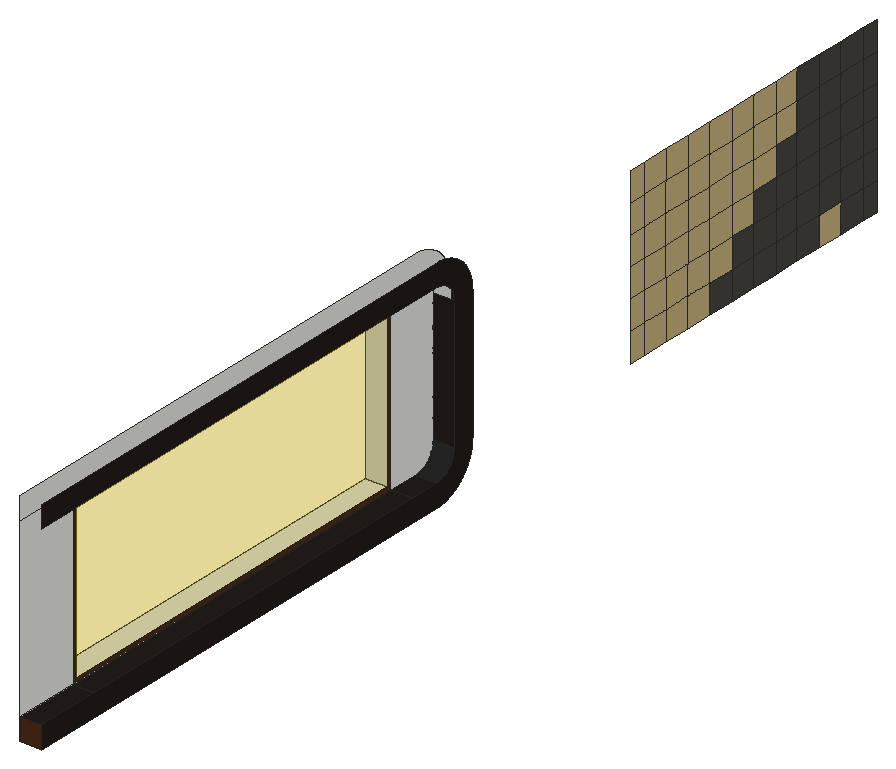
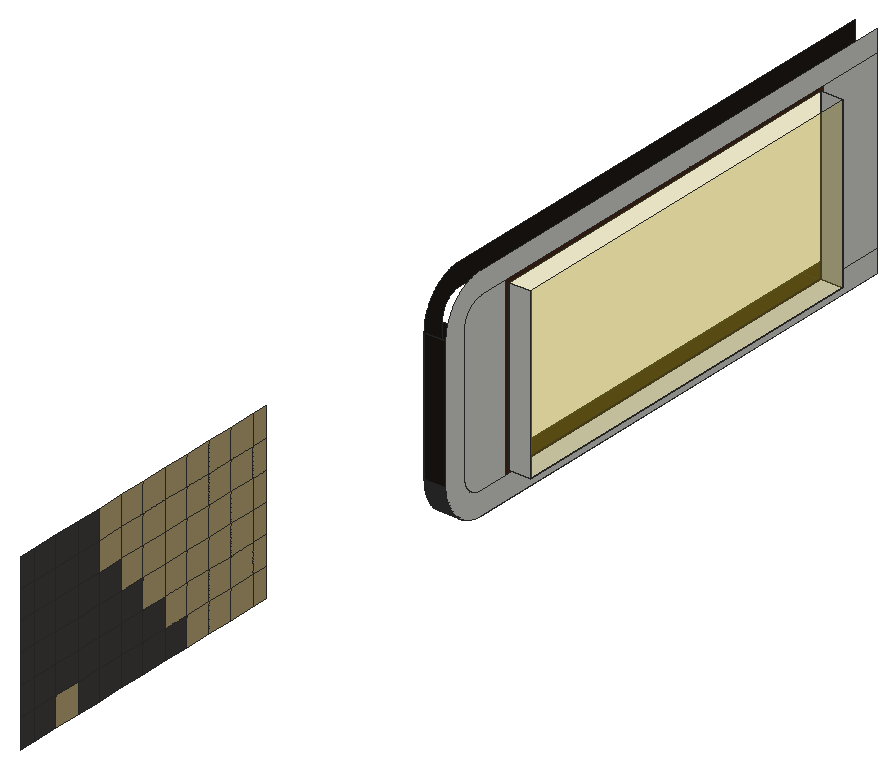
# SketchUp Ruby script. Lengths in inches.
U = 1.inch
M = Sketchup.active_model
def pt(a) = Geom::Point3d.new(a.map { |v| v * U })
def face(e, loops, mat)
  f = e.add_face(loops[0].map { |a| pt(a) })
  loops[1..].each { |l| e.add_face(l.map { |a| pt(a) }).erase! }
  f.material = f.back_material = mat if mat
  f
end
# faces: each face lists its corners as indices into pts; further lists are holes
def faces(e, pts, list, mat = nil) = list.each { |f| face(e, (f[0].is_a?(Array) ? f : [f]).map { |l| l.map { |i| pts[i] } }, mat) }
# xy, xz, yz: faces in a plane at the given z, y or x. An outline is a flat list of corners, or four numbers for a rectangle; further outlines are holes
def ring(l) = l.size == 4 ? [[l[0], l[1]], [l[2], l[1]], [l[2], l[3]], [l[0], l[3]]] : l.each_slice(2).to_a
def flat(e, list, mat, &to3) = list.each { |f| face(e, (f[0].is_a?(Array) ? f : [f]).map { |l| ring(l).map { |u, v| to3.(u, v) } }, mat) }
def xy(e, z, list, mat = nil) = flat(e, list, mat) { |x, y| [x, y, z] }
def xz(e, y, list, mat = nil) = flat(e, list, mat) { |x, z| [x, y, z] }
def yz(e, x, list, mat = nil) = flat(e, list, mat) { |y, z| [x, y, z] }
def lines(e, pts, list) = list.each { |a, b| e.add_line(pt(pts[a]), pt(pts[b])) }
# prism: a flat outline (further loops are holes) pulled along v
def prism(e, loops, v, mat = nil)
  f = face(e, loops, mat); d = Geom::Vector3d.new(v.map { |x| x * U })
  f.pushpull(f.normal.samedirection?(d) ? d.length : -d.length)
end
def box(e, o, s, mat = nil) = prism(e, [[o, [o[0] + s[0], o[1], o[2]], [o[0] + s[0], o[1] + s[1], o[2]], [o[0], o[1] + s[1], o[2]]]], [0, 0, s[2]], mat)
def at(x, y, z, deg = 0) = Geom::Transformation.translation(pt([x, y, z])) * Geom::Transformation.rotation(ORIGIN, Z_AXIS, deg.degrees)
def axes(o, x, y, z) = Geom::Transformation.new([*x, 0, *y, 0, *z, 0, *pt(o).to_a, 1])
def part(name) = M.definitions.add(name)
# library, detail: a bought-in or finely detailed component or shape, given as its bounding box
def library(name, o, s) = part(name).tap { |d| box(d.entities, o, s) }
def detail(e, o, s) = box(e.add_group.entities, o, s)
def put(e, d, t, mat = nil) = e.add_instance(d, t).tap { |i| i.material = mat if mat }
def group(e, t, mat = nil) = e.add_group.tap { |g| g.transformation = t; g.material = mat if mat }.entities
root = M.entities
M.materials.add("Glass_Basic_01").color = [255, 223, 26]
M.materials["Glass_Basic_01"].alpha = 0.25
M.materials.add("Metal_10_1K").color = [196, 175, 123]
M.materials.add("Wood_Floor_12_1K").color = [35, 29, 25]
M.materials.add("Wood_Planks_01_1K").color = [69, 67, 63]
M.materials.add("[Wood_Cherry_Original]1").color = [76, 43, 21]
xy(root,204,[[129,15,135,149.96],[129,149.96,135,150.15]],"Wood_Floor_12_1K")
xy(root,204.01,[[129,150.34,135,150.52]],"Wood_Floor_12_1K")
xy(root,210,[[129,15,135,33],[129,33,135,141.71],[129,141.71,135,149.96],[129,149.96,135,150.05],[129,150.05,135,150.15]],"Wood_Floor_12_1K")
xy(root,210.01,[[129,150.24,135,150.34]],"Wood_Floor_12_1K")
xy(root,211,[[123,34,129,140.71]])
xz(root,15,[[129,204,135,210]],"[Wood_Cherry_Original]1")
xz(root,34,[[123,211,129,257]])
xz(root,140.71,[[123,211,129,257]])
xz(root,155.95,[[129,215.625,135,215.72]],"Wood_Floor_12_1K")
xz(root,155.96,[[129,215.8125,135,215.91],[129,215.91,135,216],[129,216,135,252]],"Wood_Floor_12_1K")
xz(root,161.95,[[129,215.43,135,215.625]],"Wood_Floor_12_1K")
xz(root,161.96,[[129,215.8125,135,216],[129,216,135,252]],"Wood_Floor_12_1K")
yz(root,123,[[34,211,140.71,257]],"Glass_Basic_01")
yz(root,129,[[15,204,150.15,204,150.34,204.01,150.52,204.01,150.71,204.02,150.9,204.04,151.09,204.05,151.28,204.07,151.46,204.09,151.84,204.15,152.02,204.18,152.21,204.21,152.39,204.25,152.58,204.29,152.76,204.33,152.94,204.38,153.31,204.48,153.49,204.53,153.85,204.65,154.02,204.71,154.2,204.77,154.38,204.84,154.55,204.91,154.73,204.99,154.9,205.0625,155.07,205.14,155.24,205.22,155.41,205.31,155.57,205.39,155.74,205.48,155.91,205.58,156.07,205.67,156.55,205.97,156.7,206.08,156.86,206.18,157.16,206.4,157.3125,206.52,157.46,206.63,157.61,206.75,157.75,206.875,157.9,207,158.04,207.125,158.17,207.25,158.3125,207.38,158.44,207.51,158.58,207.65,158.71,207.79,158.84,207.92,158.96,208.0625,159.08,208.21,159.21,208.35,159.32,208.5,159.44,208.65,159.56,208.79,159.67,208.95,159.78,209.1,159.88,209.25,159.99,209.41,160.29,209.89,160.38,210.05,160.48,210.22,160.56,210.38,160.74,210.72,160.82,210.89,160.9,211.0625,160.97,211.23,161.05,211.41,161.12,211.58,161.18,211.76,161.25,211.94,161.3125,212.11,161.37,212.29,161.43,212.47,161.53,212.83,161.58,213.02,161.63,213.2,161.67,213.38,161.71,213.57,161.75,213.75,161.78,213.9375,161.8125,214.12,161.84,214.31,161.86,214.5,161.89,214.68,161.91,214.87,161.92,215.06,161.9375,215.25,161.95,215.43,161.95,215.625,161.96,215.8125,161.96,252.1875,161.95,252.375,161.95,252.57,161.9375,252.75,161.92,252.94,161.91,253.13,161.89,253.32,161.86,253.5,161.84,253.69,161.8125,253.88,161.78,254.0625,161.75,254.25,161.71,254.43,161.67,254.62,161.63,254.8,161.58,254.98,161.53,255.17,161.43,255.53,161.37,255.71,161.3125,255.89,161.25,256.06,161.18,256.24,161.12,256.42,161.05,256.59,160.97,256.77,160.9,256.9375,160.82,257.11,160.74,257.28,160.56,257.62,160.48,257.78,160.38,257.95,160.29,258.11,159.99,258.59,159.88,258.75,159.78,258.9,159.67,259.05,159.56,259.21,159.44,259.35,159.32,259.5,159.21,259.65,159.08,259.79,158.96,259.9375,158.84,260.08,158.71,260.21,158.58,260.35,158.44,260.49,158.3125,260.62,158.17,260.75,158.04,260.875,157.9,261,157.75,261.125,157.61,261.25,157.46,261.37,157.3125,261.48,157.16,261.6,156.86,261.82,156.7,261.92,156.55,262.03,156.07,262.33,155.91,262.42,155.74,262.52,155.57,262.61,155.41,262.69,155.24,262.78,155.07,262.86,154.9,262.9375,154.73,263.01,154.55,263.09,154.38,263.16,154.2,263.23,154.02,263.29,153.85,263.35,153.49,263.47,153.31,263.52,152.94,263.62,152.76,263.67,152.58,263.71,152.39,263.75,152.21,263.79,152.02,263.82,151.84,263.85,151.46,263.91,151.28,263.93,151.09,263.95,150.9,263.96,150.71,263.98,150.52,263.99,150.34,263.99,150.15,264,15,264,15,258,150.15,258,150.24,257.99,150.34,257.99,150.52,257.97,150.62,257.96,150.8,257.94,150.9,257.93,151.08,257.89,151.18,257.875,151.27,257.86,151.36,257.83,151.45,257.8125,151.54,257.79,151.72,257.73,151.8125,257.71,151.9,257.68,151.99,257.65,152.08,257.61,152.17,257.58,152.26,257.54,152.34,257.51,152.43,257.47,152.51,257.43,152.6,257.39,152.68,257.35,152.77,257.3,152.85,257.26,153.01,257.16,153.09,257.12,153.17,257.07,153.25,257.01,153.41,256.91,153.49,256.85,153.5625,256.8,153.64,256.74,153.71,256.68,153.78,256.625,153.86,256.5625,154.07,256.375,154.14,256.31,154.2,256.24,154.27,256.18,154.33,256.11,154.4,256.04,154.52,255.9,154.58,255.82,154.7,255.68,154.8125,255.53,154.87,255.45,154.97,255.29,155.03,255.21,155.08,255.13,155.17,254.97,155.22,254.89,155.26,254.81,155.31,254.72,155.35,254.64,155.39,254.55,155.43,254.47,155.47,254.38,155.5,254.3,155.54,254.21,155.6,254.03,155.64,253.94,155.67,253.85,155.69,253.76,155.75,253.58,155.79,253.4,155.82,253.31,155.83,253.22,155.87,253.03,155.89,252.9375,155.9,252.85,155.91,252.75,155.92,252.66,155.93,252.56,155.94,252.47,155.95,252.375,155.95,252.28,155.96,252.1875,155.96,215.8125,155.95,215.72,155.95,215.625,155.94,215.53,155.93,215.44,155.92,215.34,155.91,215.25,155.9,215.15,155.89,215.0625,155.87,214.97,155.83,214.78,155.82,214.69,155.79,214.6,155.75,214.42,155.69,214.24,155.67,214.15,155.64,214.06,155.6,213.97,155.54,213.79,155.5,213.7,155.47,213.62,155.43,213.53,155.39,213.45,155.35,213.36,155.31,213.28,155.26,213.19,155.22,213.11,155.17,213.03,155.08,212.87,155.03,212.79,154.97,212.71,154.87,212.55,154.8125,212.47,154.7,212.32,154.58,212.18,154.52,212.1,154.4,211.96,154.33,211.89,154.27,211.82,154.2,211.76,154.14,211.69,154.07,211.625,153.86,211.4375,153.78,211.375,153.71,211.32,153.64,211.26,153.5625,211.2,153.49,211.15,153.41,211.09,153.25,210.99,153.17,210.93,153.09,210.88,153.01,210.84,152.85,210.74,152.77,210.7,152.68,210.65,152.6,210.61,152.51,210.57,152.43,210.53,152.34,210.49,152.26,210.46,152.17,210.42,152.08,210.39,151.99,210.35,151.9,210.32,151.8125,210.29,151.72,210.27,151.54,210.21,151.45,210.1875,151.36,210.17,151.27,210.14,151.18,210.125,151.08,210.11,150.9,210.07,150.8,210.06,150.62,210.04,150.52,210.03,150.34,210.01,150.24,210.01,150.15,210,15,210],[15,210,33,258],[141.71,210,150.15,210,150.24,210.01,150.34,210.01,150.52,210.03,150.62,210.04,150.8,210.06,150.9,210.07,151.08,210.11,151.18,210.125,151.27,210.14,151.36,210.17,151.45,210.1875,151.54,210.21,151.72,210.27,151.8125,210.29,151.9,210.32,151.99,210.35,152.08,210.39,152.17,210.42,152.26,210.46,152.34,210.49,152.43,210.53,152.51,210.57,152.6,210.61,152.68,210.65,152.77,210.7,152.85,210.74,153.01,210.84,153.09,210.88,153.17,210.93,153.25,210.99,153.41,211.09,153.49,211.15,153.5625,211.2,153.64,211.26,153.71,211.32,153.78,211.375,153.86,211.4375,154.07,211.625,154.14,211.69,154.2,211.76,154.27,211.82,154.33,211.89,154.4,211.96,154.52,212.1,154.58,212.18,154.7,212.32,154.8125,212.47,154.87,212.55,154.97,212.71,155.03,212.79,155.08,212.87,155.17,213.03,155.22,213.11,155.26,213.19,155.31,213.28,155.35,213.36,155.39,213.45,155.43,213.53,155.47,213.62,155.5,213.7,155.54,213.79,155.6,213.97,155.64,214.06,155.67,214.15,155.69,214.24,155.75,214.42,155.79,214.6,155.82,214.69,155.83,214.78,155.87,214.97,155.89,215.0625,155.9,215.15,155.91,215.25,155.92,215.34,155.93,215.44,155.94,215.53,155.95,215.625,155.95,215.72,155.96,215.8125,155.96,252.1875,155.95,252.28,155.95,252.375,155.94,252.47,155.93,252.56,155.92,252.66,155.91,252.75,155.9,252.85,155.89,252.9375,155.87,253.03,155.83,253.22,155.82,253.31,155.79,253.4,155.75,253.58,155.69,253.76,155.67,253.85,155.64,253.94,155.6,254.03,155.54,254.21,155.5,254.3,155.47,254.38,155.43,254.47,155.39,254.55,155.35,254.64,155.31,254.72,155.26,254.81,155.22,254.89,155.17,254.97,155.08,255.13,155.03,255.21,154.97,255.29,154.87,255.45,154.8125,255.53,154.7,255.68,154.58,255.82,154.52,255.9,154.4,256.04,154.33,256.11,154.27,256.18,154.2,256.24,154.14,256.31,154.07,256.375,153.86,256.5625,153.78,256.625,153.71,256.68,153.64,256.74,153.5625,256.8,153.49,256.85,153.41,256.91,153.25,257.01,153.17,257.07,153.09,257.12,153.01,257.16,152.85,257.26,152.77,257.3,152.68,257.35,152.6,257.39,152.51,257.43,152.43,257.47,152.34,257.51,152.26,257.54,152.17,257.58,152.08,257.61,151.99,257.65,151.9,257.68,151.8125,257.71,151.72,257.73,151.54,257.79,151.45,257.8125,151.36,257.83,151.27,257.86,151.18,257.875,151.08,257.89,150.9,257.93,150.8,257.94,150.62,257.96,150.52,257.97,150.34,257.99,150.24,257.99,150.15,258,141.71,258]])
yz(root,129,[[34,211,140.71,257]],"Glass_Basic_01")
yz(root,129,[[[33,210,141.71,258],[34,211,140.71,257]]],"[Wood_Cherry_Original]1")
yz(root,135,[[216,210.375,220.5,218.25],[220.5,210.375,228,218.25],[228,210.375,235.5,218.25],[235.5,210.375,243,218.25],[280.5,210.375,288,218.25],
  [216,218.25,220.5,226.125],[220.5,218.25,228,226.125],[228,218.25,235.5,226.125],[235.5,218.25,243,226.125],[243,218.25,250.5,226.125],
  [216,226.125,220.5,234],[220.5,226.125,228,234],[228,226.125,235.5,234],[235.5,226.125,243,234],[243,226.125,250.5,234],
  [250.5,226.125,258,234],[216,234,220.5,241.875],[220.5,234,228,241.875],[228,234,235.5,241.875],[235.5,234,243,241.875],
  [243,234,250.5,241.875],[250.5,234,258,241.875],[258,234,265.5,241.875],[216,241.875,220.5,249.75],[220.5,241.875,228,249.75],
  [228,241.875,235.5,249.75],[235.5,241.875,243,249.75],[243,241.875,250.5,249.75],[250.5,241.875,258,249.75],[258,241.875,265.5,249.75],
  [265.5,241.875,273,249.75],[216,249.75,220.5,257.625],[220.5,249.75,228,257.625],[228,249.75,235.5,257.625],[235.5,249.75,243,257.625],
  [243,249.75,250.5,257.625],[250.5,249.75,258,257.625],[258,249.75,265.5,257.625],[265.5,249.75,273,257.625]],"Metal_10_1K")
yz(root,135,[[15,204,150.15,204,150.34,204.01,150.52,204.01,150.71,204.02,150.9,204.04,151.09,204.05,151.28,204.07,151.46,204.09,151.84,204.15,152.02,204.18,152.21,204.21,152.39,204.25,152.58,204.29,152.76,204.33,152.94,204.38,153.31,204.48,153.49,204.53,153.85,204.65,154.02,204.71,154.2,204.77,154.38,204.84,154.55,204.91,154.73,204.99,154.9,205.0625,155.07,205.14,155.24,205.22,155.41,205.31,155.57,205.39,155.74,205.48,155.91,205.58,156.07,205.67,156.55,205.97,156.7,206.08,156.86,206.18,157.16,206.4,157.3125,206.52,157.46,206.63,157.61,206.75,157.75,206.875,157.9,207,158.04,207.125,158.17,207.25,158.3125,207.38,158.44,207.51,158.58,207.65,158.71,207.79,158.84,207.92,158.96,208.0625,159.08,208.21,159.21,208.35,159.32,208.5,159.44,208.65,159.56,208.79,159.67,208.95,159.78,209.1,159.88,209.25,159.99,209.41,160.29,209.89,160.38,210.05,160.48,210.22,160.56,210.38,160.74,210.72,160.82,210.89,160.9,211.0625,160.97,211.23,161.05,211.41,161.12,211.58,161.18,211.76,161.25,211.94,161.3125,212.11,161.37,212.29,161.43,212.47,161.53,212.83,161.58,213.02,161.63,213.2,161.67,213.38,161.71,213.57,161.75,213.75,161.78,213.9375,161.8125,214.12,161.84,214.31,161.86,214.5,161.89,214.68,161.91,214.87,161.92,215.06,161.9375,215.25,161.95,215.43,161.95,215.625,161.96,215.8125,161.96,252.1875,161.95,252.375,161.95,252.57,161.9375,252.75,161.92,252.94,161.91,253.13,161.89,253.32,161.86,253.5,161.84,253.69,161.8125,253.88,161.78,254.0625,161.75,254.25,161.71,254.43,161.67,254.62,161.63,254.8,161.58,254.98,161.53,255.17,161.43,255.53,161.37,255.71,161.3125,255.89,161.25,256.06,161.18,256.24,161.12,256.42,161.05,256.59,160.97,256.77,160.9,256.9375,160.82,257.11,160.74,257.28,160.56,257.62,160.48,257.78,160.38,257.95,160.29,258.11,159.99,258.59,159.88,258.75,159.78,258.9,159.67,259.05,159.56,259.21,159.44,259.35,159.32,259.5,159.21,259.65,159.08,259.79,158.96,259.9375,158.84,260.08,158.71,260.21,158.58,260.35,158.44,260.49,158.3125,260.62,158.17,260.75,158.04,260.875,157.9,261,157.75,261.125,157.61,261.25,157.46,261.37,157.3125,261.48,157.16,261.6,156.86,261.82,156.7,261.92,156.55,262.03,156.07,262.33,155.91,262.42,155.74,262.52,155.57,262.61,155.41,262.69,155.24,262.78,155.07,262.86,154.9,262.9375,154.73,263.01,154.55,263.09,154.38,263.16,154.2,263.23,154.02,263.29,153.85,263.35,153.49,263.47,153.31,263.52,152.94,263.62,152.76,263.67,152.58,263.71,152.39,263.75,152.21,263.79,152.02,263.82,151.84,263.85,151.46,263.91,151.28,263.93,151.09,263.95,150.9,263.96,150.71,263.98,150.52,263.99,150.34,263.99,150.15,264,15,264,15,258,150.15,258,150.24,257.99,150.34,257.99,150.52,257.97,150.62,257.96,150.8,257.94,150.9,257.93,151.08,257.89,151.18,257.875,151.27,257.86,151.36,257.83,151.45,257.8125,151.54,257.79,151.72,257.73,151.8125,257.71,151.9,257.68,151.99,257.65,152.08,257.61,152.17,257.58,152.26,257.54,152.34,257.51,152.43,257.47,152.51,257.43,152.6,257.39,152.68,257.35,152.77,257.3,152.85,257.26,153.01,257.16,153.09,257.12,153.17,257.07,153.25,257.01,153.41,256.91,153.49,256.85,153.5625,256.8,153.64,256.74,153.71,256.68,153.78,256.625,153.86,256.5625,154.07,256.375,154.14,256.31,154.2,256.24,154.27,256.18,154.33,256.11,154.4,256.04,154.52,255.9,154.58,255.82,154.7,255.68,154.8125,255.53,154.87,255.45,154.97,255.29,155.03,255.21,155.08,255.13,155.17,254.97,155.22,254.89,155.26,254.81,155.31,254.72,155.35,254.64,155.39,254.55,155.43,254.47,155.47,254.38,155.5,254.3,155.54,254.21,155.6,254.03,155.64,253.94,155.67,253.85,155.69,253.76,155.75,253.58,155.79,253.4,155.82,253.31,155.83,253.22,155.87,253.03,155.89,252.9375,155.9,252.85,155.91,252.75,155.92,252.66,155.93,252.56,155.94,252.47,155.95,252.375,155.95,252.28,155.96,252.1875,155.96,215.8125,155.95,215.72,155.95,215.625,155.94,215.53,155.93,215.44,155.92,215.34,155.91,215.25,155.9,215.15,155.89,215.0625,155.87,214.97,155.83,214.78,155.82,214.69,155.79,214.6,155.75,214.42,155.69,214.24,155.67,214.15,155.64,214.06,155.6,213.97,155.54,213.79,155.5,213.7,155.47,213.62,155.43,213.53,155.39,213.45,155.35,213.36,155.31,213.28,155.26,213.19,155.22,213.11,155.17,213.03,155.08,212.87,155.03,212.79,154.97,212.71,154.87,212.55,154.8125,212.47,154.7,212.32,154.58,212.18,154.52,212.1,154.4,211.96,154.33,211.89,154.27,211.82,154.2,211.76,154.14,211.69,154.07,211.625,153.86,211.4375,153.78,211.375,153.71,211.32,153.64,211.26,153.5625,211.2,153.49,211.15,153.41,211.09,153.25,210.99,153.17,210.93,153.09,210.88,153.01,210.84,152.85,210.74,152.77,210.7,152.68,210.65,152.6,210.61,152.51,210.57,152.43,210.53,152.34,210.49,152.26,210.46,152.17,210.42,152.08,210.39,151.99,210.35,151.9,210.32,151.8125,210.29,151.72,210.27,151.54,210.21,151.45,210.1875,151.36,210.17,151.27,210.14,151.18,210.125,151.08,210.11,150.9,210.07,150.8,210.06,150.62,210.04,150.52,210.03,150.34,210.01,150.24,210.01,150.15,210,15,210]],"Wood_Floor_12_1K")
yz(root,135,[[243,210.375,250.5,218.25],[250.5,210.375,258,218.25],[258,210.375,265.5,218.25],[265.5,210.375,273,218.25],[273,210.375,280.5,218.25],
  [288,210.375,295.5,218.25],[295.5,210.375,300,218.25],[250.5,218.25,258,226.125],[258,218.25,265.5,226.125],[265.5,218.25,273,226.125],
  [273,218.25,280.5,226.125],[280.5,218.25,288,226.125],[288,218.25,295.5,226.125],[295.5,218.25,300,226.125],[258,226.125,265.5,234],
  [265.5,226.125,273,234],[273,226.125,280.5,234],[280.5,226.125,288,234],[288,226.125,295.5,234],[295.5,226.125,300,234],
  [265.5,234,273,241.875],[273,234,280.5,241.875],[280.5,234,288,241.875],[288,234,295.5,241.875],[295.5,234,300,241.875],
  [273,241.875,280.5,249.75],[280.5,241.875,288,249.75],[288,241.875,295.5,249.75],[295.5,241.875,300,249.75],[273,249.75,280.5,257.625],
  [280.5,249.75,288,257.625],[288,249.75,295.5,257.625],[295.5,249.75,300,257.625]],"Wood_Planks_01_1K")
p = [[129,150.15,204],[129,150.34,204.01],[135,150.34,204.01],[135,150.15,204],[129,150.52,204.01],[129,150.71,204.02],
  [135,150.71,204.02],[135,150.52,204.01],[129,150.9,204.04],[135,150.9,204.04],[129,151.09,204.05],[135,151.09,204.05],
  [129,151.28,204.07],[135,151.28,204.07],[129,151.46,204.09],[135,151.46,204.09],[129,151.65,204.12],[135,151.65,204.12],
  [129,151.84,204.15],[135,151.84,204.15],[129,152.02,204.18],[135,152.02,204.18],[129,152.21,204.21],[135,152.21,204.21],
  [129,152.39,204.25],[135,152.39,204.25],[129,152.58,204.29],[135,152.58,204.29],[129,152.76,204.33],[135,152.76,204.33],
  [129,152.94,204.38],[135,152.94,204.38],[129,153.125,204.43],[135,153.125,204.43],[129,153.31,204.48],[135,153.31,204.48],
  [129,153.49,204.53],[135,153.49,204.53],[129,153.67,204.59],[135,153.67,204.59],[129,153.85,204.65],[135,153.85,204.65],
  [129,154.02,204.71],[135,154.02,204.71],[129,154.2,204.77],[135,154.2,204.77],[129,154.38,204.84],[135,154.38,204.84],
  [129,154.55,204.91],[135,154.55,204.91],[129,154.73,204.99],[135,154.73,204.99],[129,154.9,205.0625],[135,154.9,205.0625],
  [129,155.07,205.14],[135,155.07,205.14],[129,155.24,205.22],[135,155.24,205.22],[129,155.41,205.31],[135,155.41,205.31],
  [129,155.57,205.39],[135,155.57,205.39],[129,155.74,205.48],[135,155.74,205.48],[129,155.91,205.58],[135,155.91,205.58],
  [129,156.07,205.67],[135,156.07,205.67],[129,156.23,205.77],[135,156.23,205.77],[129,156.39,205.87],[135,156.39,205.87],
  [129,156.55,205.97],[135,156.55,205.97],[129,156.7,206.08],[135,156.7,206.08],[129,156.86,206.18],[135,156.86,206.18],
  [129,157.01,206.29],[135,157.01,206.29],[129,157.16,206.4],[135,157.16,206.4],[129,157.3125,206.52],[135,157.3125,206.52],
  [129,157.46,206.63],[135,157.46,206.63],[129,157.61,206.75],[135,157.61,206.75],[129,157.75,206.875],[135,157.75,206.875],
  [129,157.9,207],[135,157.9,207],[129,158.04,207.125],[135,158.04,207.125],[129,158.17,207.25],[135,158.17,207.25],
  [129,158.3125,207.38],[135,158.3125,207.38],[129,158.44,207.51],[135,158.44,207.51],[129,158.58,207.65],[135,158.58,207.65],
  [129,158.71,207.79],[135,158.71,207.79],[129,158.84,207.92],[135,158.84,207.92],[129,158.96,208.0625],[135,158.96,208.0625],
  [129,159.08,208.21],[135,159.08,208.21],[129,159.21,208.35],[135,159.21,208.35],[129,159.32,208.5],[135,159.32,208.5],
  [129,159.44,208.65],[135,159.44,208.65],[129,159.56,208.79],[135,159.56,208.79],[129,159.67,208.95],[135,159.67,208.95],
  [129,159.78,209.1],[135,159.78,209.1],[129,159.88,209.25],[135,159.88,209.25],[129,159.99,209.41],[135,159.99,209.41],
  [129,160.09,209.57],[135,160.09,209.57],[129,160.19,209.73],[135,160.19,209.73],[129,160.29,209.89],[135,160.29,209.89],
  [129,160.38,210.05],[135,160.38,210.05],[129,150.24,210.01],[129,150.15,210],[135,150.15,210],[135,150.24,210.01],
  [129,150.43,210.02],[129,150.34,210.01],[135,150.34,210.01],[135,150.43,210.02],[129,150.52,210.03],[135,150.52,210.03],
  [129,150.62,210.04],[135,150.62,210.04],[129,150.71,210.05],[135,150.71,210.05],[129,150.8,210.06],[135,150.8,210.06],
  [129,150.9,210.07],[135,150.9,210.07],[129,150.99,210.09],[135,150.99,210.09],[129,151.08,210.11],[135,151.08,210.11],
  [129,151.18,210.125],[135,151.18,210.125],[129,151.27,210.14],[135,151.27,210.14],[129,151.36,210.17],[135,151.36,210.17],
  [129,160.48,210.22],[135,160.48,210.22],[129,151.45,210.1875],[135,151.45,210.1875],[129,151.54,210.21],[135,151.54,210.21],
  [129,151.63,210.24],[135,151.63,210.24],[129,151.72,210.27],[135,151.72,210.27],[129,160.56,210.38],[135,160.56,210.38],
  [129,151.8125,210.29],[135,151.8125,210.29],[129,151.9,210.32],[135,151.9,210.32],[129,151.99,210.35],[135,151.99,210.35],
  [129,152.08,210.39],[135,152.08,210.39],[129,152.17,210.42],[135,152.17,210.42],[129,152.26,210.46],[135,152.26,210.46],
  [129,160.65,210.55],[135,160.65,210.55],[129,152.34,210.49],[135,152.34,210.49],[129,152.43,210.53],[135,152.43,210.53],
  [129,152.51,210.57],[135,152.51,210.57],[129,152.6,210.61],[135,152.6,210.61],[129,152.68,210.65],[135,152.68,210.65],
  [129,160.74,210.72],[135,160.74,210.72],[129,152.77,210.7],[135,152.77,210.7],[129,152.85,210.74],[135,152.85,210.74],
  [129,152.93,210.79],[135,152.93,210.79],[129,160.82,210.89],[135,160.82,210.89],[129,153.01,210.84],[135,153.01,210.84],
  [129,153.09,210.88],[135,153.09,210.88],[129,153.17,210.93],[135,153.17,210.93],[129,153.25,210.99],[135,153.25,210.99],
  [129,160.9,211.0625],[135,160.9,211.0625],[129,153.33,211.04],[135,153.33,211.04],[129,153.41,211.09],[135,153.41,211.09],
  [129,153.49,211.15],[135,153.49,211.15],[129,153.5625,211.2],[135,153.5625,211.2],[129,160.97,211.23],[135,160.97,211.23],
  [129,153.64,211.26],[135,153.64,211.26],[129,161.05,211.41],[135,161.05,211.41],[129,153.71,211.32],[135,153.71,211.32],
  [129,153.78,211.375],[135,153.78,211.375],[129,153.86,211.4375],[135,153.86,211.4375],[129,153.93,211.5],[135,153.93,211.5],
  [129,161.12,211.58],[135,161.12,211.58],[129,154,211.5625],[135,154,211.5625],[129,154.07,211.625],[135,154.07,211.625],
  [129,154.14,211.69],[135,154.14,211.69],[129,161.18,211.76],[135,161.18,211.76],[129,154.2,211.76],[135,154.2,211.76],
  [129,154.27,211.82],[135,154.27,211.82],[129,154.33,211.89],[135,154.33,211.89],[129,161.25,211.94],[135,161.25,211.94],
  [129,154.4,211.96],[135,154.4,211.96],[129,161.3125,212.11],[135,161.3125,212.11],[129,154.46,212.03],[135,154.46,212.03],
  [129,154.52,212.1],[135,154.52,212.1],[129,154.58,212.18],[135,154.58,212.18],[129,161.37,212.29],[135,161.37,212.29],
  [129,154.64,212.25],[135,154.64,212.25],[129,154.7,212.32],[135,154.7,212.32],[129,154.76,212.4],[135,154.76,212.4],
  [129,161.43,212.47],[135,161.43,212.47],[129,154.8125,212.47],[135,154.8125,212.47],[129,154.87,212.55],[135,154.87,212.55],
  [129,154.92,212.63],[135,154.92,212.63],[129,161.48,212.65],[135,161.48,212.65],[129,154.97,212.71],[135,154.97,212.71],
  [129,155.03,212.79],[135,155.03,212.79],[129,161.53,212.83],[135,161.53,212.83],[129,155.08,212.87],[135,155.08,212.87],
  [129,161.58,213.02],[135,161.58,213.02],[129,155.125,212.95],[135,155.125,212.95],[129,155.17,213.03],[135,155.17,213.03],
  [129,155.22,213.11],[135,155.22,213.11],[129,161.63,213.2],[135,161.63,213.2],[129,155.26,213.19],[135,155.26,213.19],
  [129,155.31,213.28],[135,155.31,213.28],[129,161.67,213.38],[135,161.67,213.38],[129,155.35,213.36],[135,155.35,213.36],
  [129,155.39,213.45],[135,155.39,213.45],[129,155.43,213.53],[135,155.43,213.53],[129,161.71,213.57],[135,161.71,213.57],
  [129,155.47,213.62],[135,155.47,213.62],[129,155.5,213.7],[135,155.5,213.7],[129,161.75,213.75],[135,161.75,213.75],
  [129,155.54,213.79],[135,155.54,213.79],[129,155.57,213.88],[135,155.57,213.88],[129,161.78,213.9375],[135,161.78,213.9375],
  [129,155.6,213.97],[135,155.6,213.97],[129,161.8125,214.12],[135,161.8125,214.12],[129,155.64,214.06],[135,155.64,214.06],
  [129,155.67,214.15],[135,155.67,214.15],[129,155.69,214.24],[135,155.69,214.24],[129,161.84,214.31],[135,161.84,214.31],
  [129,155.72,214.33],[135,155.72,214.33],[129,155.75,214.42],[135,155.75,214.42],[129,161.86,214.5],[135,161.86,214.5],
  [129,155.77,214.51],[135,155.77,214.51],[129,155.79,214.6],[135,155.79,214.6],[129,161.89,214.68],[135,161.89,214.68],
  [129,155.82,214.69],[135,155.82,214.69],[129,155.83,214.78],[135,155.83,214.78],[129,161.91,214.87],[135,161.91,214.87],
  [129,155.85,214.875],[135,155.85,214.875],[129,155.87,214.97],[135,155.87,214.97],[129,161.92,215.06],[135,161.92,215.06],
  [129,155.89,215.0625],[135,155.89,215.0625],[129,155.9,215.15],[135,155.9,215.15],[129,161.9375,215.25],[135,161.9375,215.25],
  [129,155.91,215.25],[135,155.91,215.25],[129,155.92,215.34],[135,155.92,215.34],[129,161.95,215.43],[135,161.95,215.43],
  [129,155.93,215.44],[135,155.93,215.44],[129,155.94,215.53],[135,155.94,215.53],[129,155.95,215.625],[135,155.95,215.625],
  [129,161.95,215.625],[129,161.96,215.8125],[135,161.96,215.8125],[135,161.95,215.625],[129,155.96,215.8125],[129,155.95,215.72],
  [135,155.95,215.72],[135,155.96,215.8125]]
faces(root,p,[[0,1,2,3],[4,5,6,7],[5,8,9,6],[8,10,11,9],[10,12,13,11],[12,14,15,13],[14,16,17,15],[16,18,19,17],
  [18,20,21,19],[20,22,23,21],[22,24,25,23],[24,26,27,25],[26,28,29,27],[28,30,31,29],[30,32,33,31],[32,34,35,33],
  [34,36,37,35],[36,38,39,37],[38,40,41,39],[40,42,43,41],[42,44,45,43],[44,46,47,45],[46,48,49,47],[48,50,51,49],
  [50,52,53,51],[52,54,55,53],[54,56,57,55],[56,58,59,57],[58,60,61,59],[60,62,63,61],[62,64,65,63],[64,66,67,65],
  [66,68,69,67],[68,70,71,69],[70,72,73,71],[72,74,75,73],[74,76,77,75],[76,78,79,77],[78,80,81,79],[80,82,83,81],
  [82,84,85,83],[84,86,87,85],[86,88,89,87],[88,90,91,89],[90,92,93,91],[92,94,95,93],[94,96,97,95],[96,98,99,97],
  [98,100,101,99],[100,102,103,101],[102,104,105,103],[104,106,107,105],[106,108,109,107],[108,110,111,109],[110,112,113,111],[112,114,115,113],
  [114,116,117,115],[116,118,119,117],[118,120,121,119],[120,122,123,121],[122,124,125,123],[124,126,127,125],[126,128,129,127],[128,130,131,129],
  [130,132,133,131],[134,135,136,137],[138,139,140,141],[142,138,141,143],[144,142,143,145],[146,144,145,147],[148,146,147,149],[150,148,149,151],
  [152,150,151,153],[154,152,153,155],[156,154,155,157],[158,156,157,159],[160,158,159,161],[132,162,163,133],[164,160,161,165],[166,164,165,167],
  [168,166,167,169],[170,168,169,171],[162,172,173,163],[174,170,171,175],[176,174,175,177],[178,176,177,179],[180,178,179,181],[182,180,181,183],
  [184,182,183,185],[172,186,187,173],[188,184,185,189],[190,188,189,191],[192,190,191,193],[194,192,193,195],[196,194,195,197],[186,198,199,187],
  [200,196,197,201],[202,200,201,203],[204,202,203,205],[198,206,207,199],[208,204,205,209],[210,208,209,211],[212,210,211,213],[214,212,213,215],
  [206,216,217,207],[218,214,215,219],[220,218,219,221],[222,220,221,223],[224,222,223,225],[216,226,227,217],[228,224,225,229],[226,230,231,227],
  [232,228,229,233],[234,232,233,235],[236,234,235,237],[238,236,237,239],[230,240,241,231],[242,238,239,243],[244,242,243,245],[246,244,245,247],
  [240,248,249,241],[250,246,247,251],[252,250,251,253],[254,252,253,255],[248,256,257,249],[258,254,255,259],[256,260,261,257],[262,258,259,263],
  [264,262,263,265],[266,264,265,267],[260,268,269,261],[270,266,267,271],[272,270,271,273],[274,272,273,275],[268,276,277,269],[278,274,275,279],
  [280,278,279,281],[282,280,281,283],[276,284,285,277],[286,282,283,287],[288,286,287,289],[284,290,291,285],[292,288,289,293],[290,294,295,291],
  [296,292,293,297],[298,296,297,299],[300,298,299,301],[294,302,303,295],[304,300,301,305],[306,304,305,307],[302,308,309,303],[310,306,307,311],
  [312,310,311,313],[314,312,313,315],[308,316,317,309],[318,314,315,319],[320,318,319,321],[316,322,323,317],[324,320,321,325],[326,324,325,327],
  [322,328,329,323],[330,326,327,331],[328,332,333,329],[334,330,331,335],[336,334,335,337],[338,336,337,339],[332,340,341,333],[342,338,339,343],
  [344,342,343,345],[340,346,347,341],[348,344,345,349],[350,348,349,351],[346,352,353,347],[354,350,351,355],[356,354,355,357],[352,358,359,353],
  [360,356,357,361],[362,360,361,363],[358,364,365,359],[366,362,363,367],[368,366,367,369],[364,370,371,365],[372,368,369,373],[374,372,373,375],
  [370,376,377,371],[378,374,375,379],[380,378,379,381],[382,380,381,383],[384,385,386,387],[388,389,390,391]],"Wood_Floor_12_1K")
